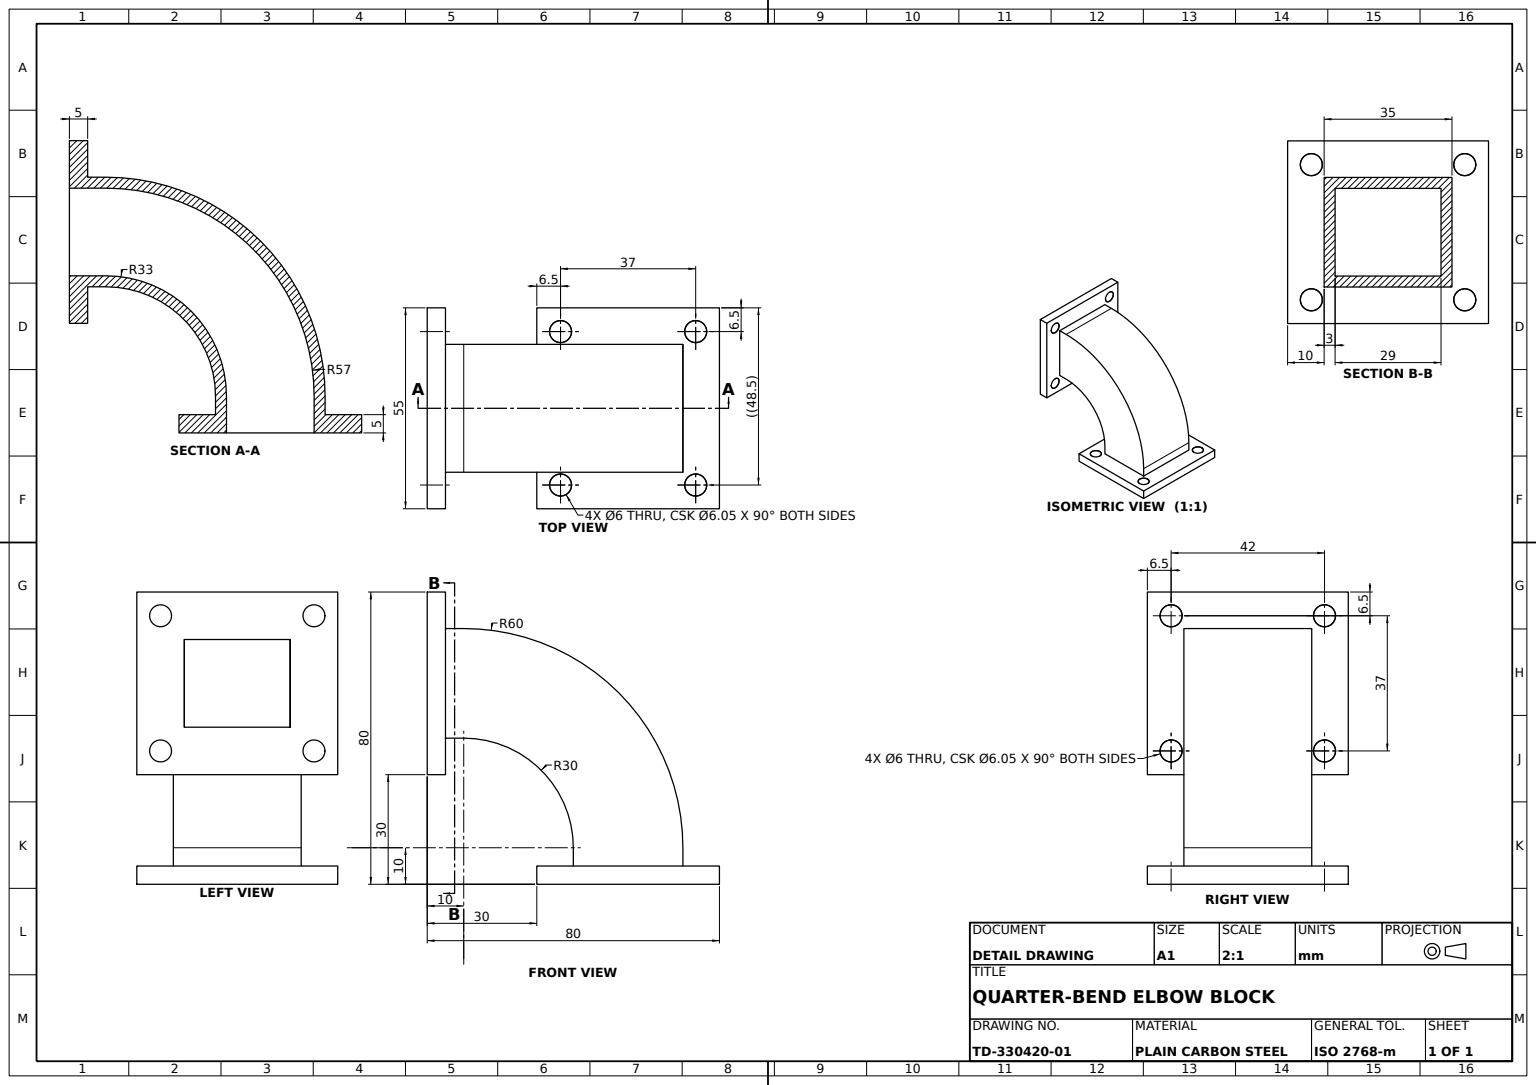
solid
v1 (30,-55,-27.5)
v2 (30,-50,-27.5)
e1 v1 v2 LINE
v3 (80,-50,-27.5)
e2 v2 v3 LINE
v4 (80,-55,-27.5)
e3 v3 v4 LINE
e4 v4 v1 LINE
face PLANE(AX(P(0,0,-27.5),D(0,0,1),D(1,0,0))) rev [e1 e2 e3 e4]
v5 (36.5,-55,18)
v6 (36.5,-55,24)
e5 v5 v6 CIRCLE(AX(P(36.5,-55,21),D(0,1,0),D(0,0,1)),3)
e6 v6 v5 CIRCLE(AX(P(36.5,-55,21),D(0,1,0),D(0,0,1)),3)
v7 (80,-55,27.5)
v8 (30,-55,27.5)
e7 v7 v8 LINE
e8 v1 v8 LINE
e9 v4 v7 LINE
v9 (73.5,-55,18)
v10 (73.5,-55,24)
e10 v9 v10 CIRCLE(AX(P(73.5,-55,21),D(0,1,0),D(0,0,1)),3)
e11 v10 v9 CIRCLE(AX(P(73.5,-55,21),D(0,1,0),D(0,0,1)),3)
v11 (36.5,-55,-18)
v12 (36.5,-55,-24)
e12 v11 v12 CIRCLE(AX(P(36.5,-55,-21),D(0,1,0),D(0,0,1)),3)
e13 v12 v11 CIRCLE(AX(P(36.5,-55,-21),D(0,1,0),D(0,0,1)),3)
v13 (73.5,-55,-24)
v14 (73.5,-55,-18)
e14 v13 v14 CIRCLE(AX(P(73.5,-55,-21),D(0,1,0),D(0,0,1)),3)
e15 v14 v13 CIRCLE(AX(P(73.5,-55,-21),D(0,1,0),D(0,0,1)),3)
v15 (67,-55,14.5)
v16 (43,-55,14.5)
e16 v15 v16 LINE
v17 (67,-55,-14.5)
e17 v15 v17 LINE
v18 (43,-55,-14.5)
e18 v17 v18 LINE
e19 v16 v18 LINE
face PLANE(AX(P(0,-55,-27.5),D(0,1,0),D(-1,0,0))) rev [e5 e6] [e7 -e8 -e4 e9] [e10 e11] [e12 e13] [e14 e15] [-e16 e17 e18 -e19]
v19 (36.5,-50.025,-24)
v20 (36.5,-50.025,-18)
e20 v19 v20 CIRCLE(AX(P(36.5,-50.025,-21),D(0,1,0),D(0,0,1)),3)
v21 (36.5,-50,-24.025)
e21 v19 v21 LINE
v22 (36.5,-50,-17.975)
e22 v21 v22 CIRCLE(AX(P(36.5,-50,-21),D(0,1,0),D(0,0,1)),3.025)
e23 v20 v22 LINE
face CONE(AX(P(36.5,-50,-21),D(0,1,0),D(0,0,1)),3.025,0.785398163) rev [-e20 e21 e22 -e23]
v23 (5,18.5,17.975)
v24 (5,18.5,24.025)
e24 v23 v24 CIRCLE(AX(P(5,18.5,21),D(1,0,0),D(0,0,-1)),3.025)
e25 v24 v23 CIRCLE(AX(P(5,18.5,21),D(1,0,0),D(0,0,-1)),3.025)
v25 (5,-18.5,17.975)
v26 (5,-18.5,24.025)
e26 v25 v26 CIRCLE(AX(P(5,-18.5,21),D(1,0,0),D(0,0,-1)),3.025)
e27 v26 v25 CIRCLE(AX(P(5,-18.5,21),D(1,0,0),D(0,0,-1)),3.025)
v27 (5,-25,27.5)
v28 (5,25,27.5)
e28 v27 v28 LINE
v29 (5,-25,-27.5)
e29 v29 v27 LINE
v30 (5,25,-27.5)
e30 v29 v30 LINE
e31 v30 v28 LINE
v31 (5,15,-17.5)
v32 (5,15,17.5)
e32 v31 v32 LINE
v33 (5,-15,-17.5)
e33 v33 v31 LINE
v34 (5,-15,17.5)
e34 v33 v34 LINE
e35 v34 v32 LINE
v35 (5,-18.5,-17.975)
v36 (5,-18.5,-24.025)
e36 v35 v36 CIRCLE(AX(P(5,-18.5,-21),D(1,0,0),D(0,0,-1)),3.025)
e37 v36 v35 CIRCLE(AX(P(5,-18.5,-21),D(1,0,0),D(0,0,-1)),3.025)
v37 (5,18.5,-17.975)
v38 (5,18.5,-24.025)
e38 v37 v38 CIRCLE(AX(P(5,18.5,-21),D(1,0,0),D(0,0,-1)),3.025)
e39 v38 v37 CIRCLE(AX(P(5,18.5,-21),D(1,0,0),D(0,0,-1)),3.025)
face PLANE(AX(P(5,0,-27.5),D(1,0,0),D(0,1,0))) [-e24 -e25] [-e26 -e27] [-e28 -e29 e30 e31] [-e32 -e33 e34 e35] [-e36 -e37] [-e38 -e39]
v39 (0,25,-27.5)
e40 v30 v39 LINE
v40 (0,25,27.5)
e41 v39 v40 LINE
e42 v28 v40 LINE
face PLANE(AX(P(0,25,-27.5),D(0,1,0),D(-1,0,0))) [-e31 e40 e41 -e42]
v41 (0,18.5,24)
v42 (4.975,18.5,24)
e43 v41 v42 LINE
v43 (4.975,18.5,18)
e44 v42 v43 CIRCLE(AX(P(4.975,18.5,21),D(1,0,0),D(0,0,-1)),3)
v44 (0,18.5,18)
e45 v44 v43 LINE
e46 v41 v44 CIRCLE(AX(P(0,18.5,21),D(1,0,0),D(0,0,-1)),3)
face CYL(AX(P(5,18.5,21),D(1,0,0),D(0,0,-1)),3) rev [e43 e44 -e45 -e46]
v45 (80,-50,27.5)
e47 v45 v7 LINE
v46 (30,-50,27.5)
e48 v46 v45 LINE
e49 v8 v46 LINE
face PLANE(AX(P(0,0,27.5),D(0,0,1),D(1,0,0))) [-e47 -e48 -e49 -e7]
v47 (0,-18.5,-18)
v48 (4.975,-18.5,-18)
e50 v47 v48 LINE
v49 (0,-18.5,-24)
e51 v49 v47 CIRCLE(AX(P(0,-18.5,-21),D(1,0,0),D(0,0,-1)),3)
v50 (4.975,-18.5,-24)
e52 v49 v50 LINE
e53 v50 v48 CIRCLE(AX(P(4.975,-18.5,-21),D(1,0,0),D(0,0,-1)),3)
face CYL(AX(P(5,-18.5,-21),D(1,0,0),D(0,0,-1)),3) rev [-e50 -e51 e52 e53]
v51 (43,-45,14.5)
v52 (10,-12,14.5)
e54 v51 v52 CIRCLE(AX(P(10,-45,14.5),D(0,0,1),D(1,0,0)),33)
v53 (43,-45,-14.5)
e55 v51 v53 LINE
v54 (10,-12,-14.5)
e56 v53 v54 CIRCLE(AX(P(10,-45,-14.5),D(0,0,1),D(1,0,0)),33)
e57 v52 v54 LINE
face CYL(AX(P(10,-45,14.5),D(0,0,-1),D(-1,0,0)),33) [-e54 e55 e56 -e57]
e58 v42 v24 LINE
e59 v43 v23 LINE
face CONE(AX(P(5,18.5,21),D(1,0,0),D(0,0,-1)),3.025,0.785398163) rev [-e44 e58 e25 -e59]
v55 (10,15,-17.5)
e60 v31 v55 LINE
v56 (10,15,17.5)
e61 v32 v56 LINE
e62 v55 v56 LINE
face PLANE(AX(P(0,15,-17.5),D(0,-1,0),D(0,0,-1))) rev [-e60 e32 e61 -e62]
v57 (40,-50,-17.5)
v58 (40,-45,-17.5)
e63 v57 v58 LINE
v59 (40,-50,17.5)
e64 v57 v59 LINE
v60 (40,-45,17.5)
e65 v59 v60 LINE
e66 v58 v60 LINE
face PLANE(AX(P(40,0,-17.5),D(1,0,0),D(0,0,-1))) rev [-e63 e64 e65 -e66]
v61 (4.975,-18.5,24)
v62 (4.975,-18.5,18)
e67 v61 v62 CIRCLE(AX(P(4.975,-18.5,21),D(1,0,0),D(0,0,-1)),3)
v63 (0,-18.5,18)
e68 v63 v62 LINE
v64 (0,-18.5,24)
e69 v64 v63 CIRCLE(AX(P(0,-18.5,21),D(1,0,0),D(0,0,-1)),3)
e70 v64 v61 LINE
face CYL(AX(P(5,-18.5,21),D(1,0,0),D(0,0,-1)),3) rev [e67 -e68 -e69 e70]
e71 v16 v51 LINE
v65 (0,-12,14.5)
e72 v65 v52 LINE
v66 (0,12,14.5)
e73 v66 v65 LINE
v67 (10,12,14.5)
e74 v66 v67 LINE
v68 (67,-45,14.5)
e75 v68 v67 CIRCLE(AX(P(10,-45,14.5),D(0,0,1),D(1,0,0)),57)
e76 v15 v68 LINE
face PLANE(AX(P(0,0,14.5),D(0,0,1),D(1,0,0))) rev [e16 e71 e54 -e72 -e73 e74 -e75 -e76]
v69 (67,-45,-14.5)
e77 v17 v69 LINE
e78 v68 v69 LINE
face PLANE(AX(P(67,0,14.5),D(-1,0,0),D(0,-1,0))) [-e77 -e17 e76 e78]
v70 (4.975,18.5,-18)
v71 (4.975,18.5,-24)
e79 v70 v71 CIRCLE(AX(P(4.975,18.5,-21),D(1,0,0),D(0,0,-1)),3)
v72 (0,18.5,-24)
e80 v72 v71 LINE
v73 (0,18.5,-18)
e81 v73 v72 CIRCLE(AX(P(0,18.5,-21),D(1,0,0),D(0,0,-1)),3)
e82 v73 v70 LINE
face CYL(AX(P(5,18.5,-21),D(1,0,0),D(0,0,-1)),3) rev [e79 -e80 -e81 e82]
v74 (36.5,-50,24.025)
v75 (36.5,-50,17.975)
e83 v74 v75 CIRCLE(AX(P(36.5,-50,21),D(0,1,0),D(0,0,1)),3.025)
v76 (36.5,-50.025,18)
e84 v76 v75 LINE
v77 (36.5,-50.025,24)
e85 v77 v76 CIRCLE(AX(P(36.5,-50.025,21),D(0,1,0),D(0,0,1)),3)
e86 v77 v74 LINE
face CONE(AX(P(36.5,-50,21),D(0,1,0),D(0,0,1)),3.025,0.785398163) rev [e83 -e84 -e85 e86]
e87 v62 v61 CIRCLE(AX(P(4.975,-18.5,21),D(1,0,0),D(0,0,-1)),3)
e88 v63 v64 CIRCLE(AX(P(0,-18.5,21),D(1,0,0),D(0,0,-1)),3)
face CYL(AX(P(5,-18.5,21),D(1,0,0),D(0,0,-1)),3) rev [e87 -e70 -e88 e68]
e89 v61 v26 LINE
e90 v62 v25 LINE
face CONE(AX(P(5,-18.5,21),D(1,0,0),D(0,0,-1)),3.025,0.785398163) rev [e26 -e89 -e87 e90]
e91 v71 v38 LINE
e92 v70 v37 LINE
face CONE(AX(P(5,18.5,-21),D(1,0,0),D(0,0,-1)),3.025,0.785398163) rev [e38 -e91 -e79 e92]
v78 (10,-15,17.5)
e93 v34 v78 LINE
e94 v60 v78 CIRCLE(AX(P(10,-45,17.5),D(0,0,1),D(1,0,0)),30)
v79 (70,-50,17.5)
e95 v59 v79 LINE
v80 (70,-45,17.5)
e96 v79 v80 LINE
e97 v80 v56 CIRCLE(AX(P(10,-45,17.5),D(0,0,1),D(1,0,0)),60)
face PLANE(AX(P(0,0,17.5),D(0,0,1),D(1,0,0))) [-e35 e93 -e94 -e65 e95 e96 e97 -e61]
e98 v12 v19 LINE
e99 v11 v20 LINE
face CYL(AX(P(36.5,-50,-21),D(0,1,0),D(0,0,1)),3) rev [-e13 e98 e20 -e99]
e100 v6 v77 LINE
e101 v5 v76 LINE
face CYL(AX(P(36.5,-50,21),D(0,1,0),D(0,0,1)),3) rev [e100 e85 -e101 -e6]
e102 v43 v42 CIRCLE(AX(P(4.975,18.5,21),D(1,0,0),D(0,0,-1)),3)
face CONE(AX(P(5,18.5,21),D(1,0,0),D(0,0,-1)),3.025,0.785398163) rev [e59 e24 -e58 -e102]
v81 (10,-15,-17.5)
e103 v81 v78 LINE
e104 v58 v81 CIRCLE(AX(P(10,-45,-17.5),D(0,0,1),D(1,0,0)),30)
face CYL(AX(P(10,-45,-17.5),D(0,0,1),D(1,0,0)),30) rev [e66 e94 -e103 -e104]
e105 v3 v45 LINE
e106 v2 v46 LINE
e107 v75 v74 CIRCLE(AX(P(36.5,-50,21),D(0,1,0),D(0,0,1)),3.025)
v82 (70,-50,-17.5)
e108 v57 v82 LINE
e109 v82 v79 LINE
v83 (73.5,-50,24.025)
v84 (73.5,-50,17.975)
e110 v83 v84 CIRCLE(AX(P(73.5,-50,21),D(0,1,0),D(0,0,1)),3.025)
e111 v84 v83 CIRCLE(AX(P(73.5,-50,21),D(0,1,0),D(0,0,1)),3.025)
v85 (73.5,-50,-24.025)
v86 (73.5,-50,-17.975)
e112 v85 v86 CIRCLE(AX(P(73.5,-50,-21),D(0,1,0),D(0,0,1)),3.025)
e113 v86 v85 CIRCLE(AX(P(73.5,-50,-21),D(0,1,0),D(0,0,1)),3.025)
e114 v22 v21 CIRCLE(AX(P(36.5,-50,-21),D(0,1,0),D(0,0,1)),3.025)
face PLANE(AX(P(0,-50,-27.5),D(0,-1,0),D(1,0,0))) rev [e48 -e105 -e2 e106] [-e107 -e83] [-e95 -e64 e108 e109] [-e110 -e111] [-e112 -e113] [-e22 -e114]
v87 (10,12,-14.5)
e115 v69 v87 CIRCLE(AX(P(10,-45,-14.5),D(0,0,1),D(1,0,0)),57)
v88 (0,12,-14.5)
e116 v88 v87 LINE
v89 (0,-12,-14.5)
e117 v88 v89 LINE
e118 v89 v54 LINE
e119 v18 v53 LINE
face PLANE(AX(P(0,0,-14.5),D(0,0,1),D(1,0,0))) [e77 e115 -e116 e117 e118 -e56 -e119 -e18]
e120 v44 v41 CIRCLE(AX(P(0,18.5,21),D(1,0,0),D(0,0,-1)),3)
face CYL(AX(P(5,18.5,21),D(1,0,0),D(0,0,-1)),3) rev [-e120 e45 e102 -e43]
face CONE(AX(P(5,-18.5,21),D(1,0,0),D(0,0,-1)),3.025,0.785398163) rev [e27 -e90 -e67 e89]
e121 v71 v70 CIRCLE(AX(P(4.975,18.5,-21),D(1,0,0),D(0,0,-1)),3)
face CONE(AX(P(5,18.5,-21),D(1,0,0),D(0,0,-1)),3.025,0.785398163) rev [-e121 e91 e39 -e92]
v90 (73.5,-50.025,18)
v91 (73.5,-50.025,24)
e122 v90 v91 CIRCLE(AX(P(73.5,-50.025,21),D(0,1,0),D(0,0,1)),3)
e123 v10 v91 LINE
e124 v9 v90 LINE
face CYL(AX(P(73.5,-50,21),D(0,1,0),D(0,0,1)),3) rev [e122 -e123 -e10 e124]
v92 (73.5,-50.025,-18)
e125 v92 v86 LINE
v93 (73.5,-50.025,-24)
e126 v93 v92 CIRCLE(AX(P(73.5,-50.025,-21),D(0,1,0),D(0,0,1)),3)
e127 v93 v85 LINE
face CONE(AX(P(73.5,-50,-21),D(0,1,0),D(0,0,1)),3.025,0.785398163) rev [-e125 -e126 e127 e112]
face PLANE(AX(P(80,0,-27.5),D(-1,0,0),D(0,-1,0))) rev [-e3 e105 e47 -e9]
e128 v20 v19 CIRCLE(AX(P(36.5,-50.025,-21),D(0,1,0),D(0,0,1)),3)
face CYL(AX(P(36.5,-50,-21),D(0,1,0),D(0,0,1)),3) rev [e128 -e98 -e12 e99]
v94 (0,-25,27.5)
e129 v40 v94 LINE
e130 v27 v94 LINE
face PLANE(AX(P(0,0,27.5),D(0,0,1),D(1,0,0))) [e129 -e130 e28 e42]
e131 v91 v83 LINE
e132 v90 v84 LINE
face CONE(AX(P(73.5,-50,21),D(0,1,0),D(0,0,1)),3.025,0.785398163) rev [-e131 -e122 e132 e111]
v95 (70,-45,-17.5)
e133 v95 v55 CIRCLE(AX(P(10,-45,-17.5),D(0,0,1),D(1,0,0)),60)
e134 v95 v80 LINE
face CYL(AX(P(10,-45,-17.5),D(0,0,1),D(1,0,0)),60) [e133 e62 -e97 -e134]
v96 (0,-25,-27.5)
e135 v29 v96 LINE
e136 v96 v94 LINE
face PLANE(AX(P(0,-25,-27.5),D(0,1,0),D(-1,0,0))) rev [-e135 e29 e130 -e136]
e137 v14 v92 LINE
e138 v13 v93 LINE
face CYL(AX(P(73.5,-50,-21),D(0,1,0),D(0,0,1)),3) rev [e126 -e137 -e14 e138]
e139 v65 v89 LINE
e140 v66 v88 LINE
e141 v47 v49 CIRCLE(AX(P(0,-18.5,-21),D(1,0,0),D(0,0,-1)),3)
e142 v72 v73 CIRCLE(AX(P(0,18.5,-21),D(1,0,0),D(0,0,-1)),3)
e143 v39 v96 LINE
face PLANE(AX(P(0,0,-27.5),D(-1,0,0),D(0,-1,0))) [e139 -e117 -e140 e73] [e46 e120] [e88 e69] [e141 e51] [e81 e142] [-e129 -e41 e143 e136]
e144 v33 v81 LINE
face PLANE(AX(P(0,-15,-17.5),D(0,-1,0),D(1,0,0))) [e144 e103 -e93 -e34]
face PLANE(AX(P(0,-12,14.5),D(0,1,0),D(-1,0,0))) [-e139 e72 e57 -e118]
face CONE(AX(P(36.5,-50,-21),D(0,1,0),D(0,0,1)),3.025,0.785398163) rev [e114 -e21 -e128 e23]
face PLANE(AX(P(43,0,14.5),D(-1,0,0),D(0,-1,0))) rev [e19 e119 -e55 -e71]
e145 v91 v90 CIRCLE(AX(P(73.5,-50.025,21),D(0,1,0),D(0,0,1)),3)
face CYL(AX(P(73.5,-50,21),D(0,1,0),D(0,0,1)),3) rev [-e11 e123 e145 -e124]
face PLANE(AX(P(30,0,-27.5),D(1,0,0),D(0,0,-1))) rev [e8 e49 -e106 -e1]
e146 v92 v93 CIRCLE(AX(P(73.5,-50.025,-21),D(0,1,0),D(0,0,1)),3)
face CYL(AX(P(73.5,-50,-21),D(0,1,0),D(0,0,1)),3) rev [-e15 e137 e146 -e138]
e147 v67 v87 LINE
face CYL(AX(P(10,-45,14.5),D(0,0,-1),D(-1,0,0)),57) rev [e147 -e115 -e78 e75]
e148 v76 v77 CIRCLE(AX(P(36.5,-50.025,21),D(0,1,0),D(0,0,1)),3)
face CONE(AX(P(36.5,-50,21),D(0,1,0),D(0,0,1)),3.025,0.785398163) rev [-e86 -e148 e84 e107]
face CYL(AX(P(36.5,-50,21),D(0,1,0),D(0,0,1)),3) rev [-e5 e101 e148 -e100]
e149 v48 v35 LINE
e150 v50 v36 LINE
face CONE(AX(P(5,-18.5,-21),D(1,0,0),D(0,0,-1)),3.025,0.785398163) rev [-e149 -e53 e150 e37]
e151 v82 v95 LINE
face PLANE(AX(P(0,0,-17.5),D(0,0,1),D(1,0,0))) rev [-e144 e33 e60 -e133 -e151 -e108 e63 e104]
face PLANE(AX(P(0,12,14.5),D(0,1,0),D(-1,0,0))) rev [e116 -e147 -e74 e140]
e152 v48 v50 CIRCLE(AX(P(4.975,-18.5,-21),D(1,0,0),D(0,0,-1)),3)
face CYL(AX(P(5,-18.5,-21),D(1,0,0),D(0,0,-1)),3) rev [e50 e152 -e52 -e141]
face PLANE(AX(P(70,0,-17.5),D(1,0,0),D(0,1,0))) [e134 -e96 -e109 e151]
face CONE(AX(P(5,-18.5,-21),D(1,0,0),D(0,0,-1)),3.025,0.785398163) rev [-e150 -e152 e149 e36]
face CONE(AX(P(73.5,-50,-21),D(0,1,0),D(0,0,1)),3.025,0.785398163) rev [e125 e113 -e127 -e146]
face PLANE(AX(P(0,0,-27.5),D(0,0,1),D(1,0,0))) rev [e135 -e143 -e40 -e30]
face CONE(AX(P(73.5,-50,21),D(0,1,0),D(0,0,1)),3.025,0.785398163) rev [-e132 -e145 e131 e110]
face CYL(AX(P(5,18.5,-21),D(1,0,0),D(0,0,-1)),3) rev [-e142 e80 e121 -e82]
